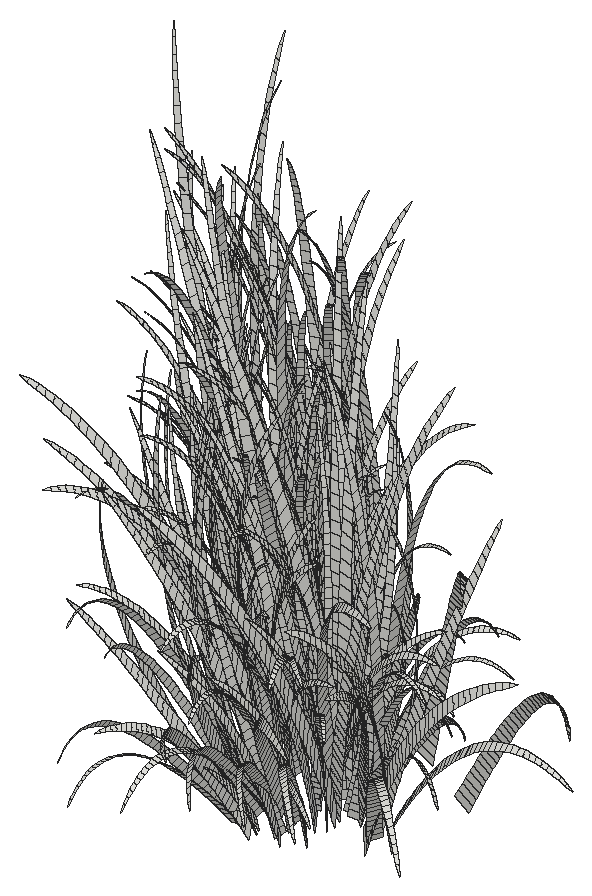
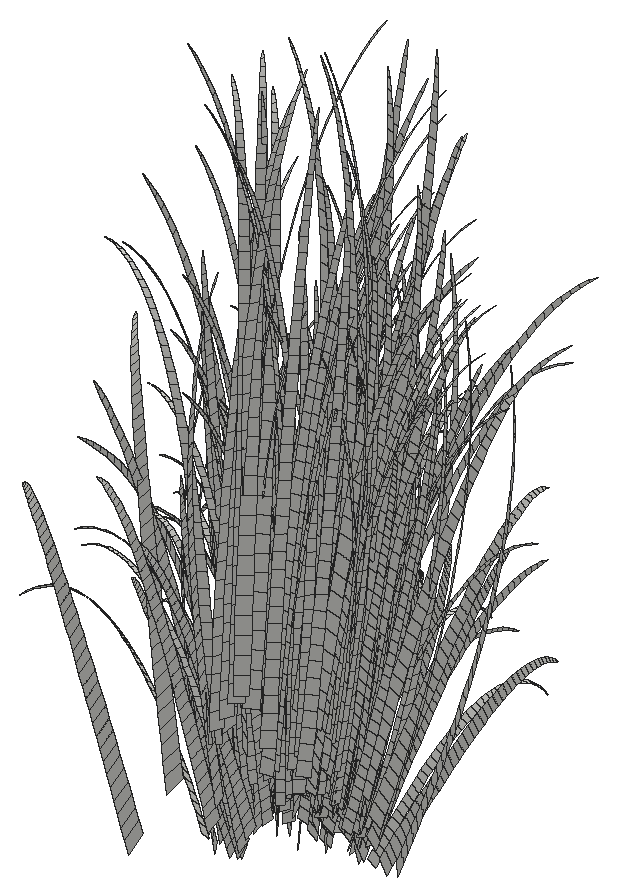
# SketchUp Ruby script. Lengths in inches.
U = 1.inch
M = Sketchup.active_model
def pt(a) = Geom::Point3d.new(a.map { |v| v * U })
def face(e, loops, mat)
  f = e.add_face(loops[0].map { |a| pt(a) })
  loops[1..].each { |l| e.add_face(l.map { |a| pt(a) }).erase! }
  f.material = f.back_material = mat if mat
  f
end
# faces: each face lists its corners as indices into pts; further lists are holes
def faces(e, pts, list, mat = nil) = list.each { |f| face(e, (f[0].is_a?(Array) ? f : [f]).map { |l| l.map { |i| pts[i] } }, mat) }
# xy, xz, yz: faces in a plane at the given z, y or x. An outline is a flat list of corners, or four numbers for a rectangle; further outlines are holes
def ring(l) = l.size == 4 ? [[l[0], l[1]], [l[2], l[1]], [l[2], l[3]], [l[0], l[3]]] : l.each_slice(2).to_a
def flat(e, list, mat, &to3) = list.each { |f| face(e, (f[0].is_a?(Array) ? f : [f]).map { |l| ring(l).map { |u, v| to3.(u, v) } }, mat) }
def xy(e, z, list, mat = nil) = flat(e, list, mat) { |x, y| [x, y, z] }
def xz(e, y, list, mat = nil) = flat(e, list, mat) { |x, z| [x, y, z] }
def yz(e, x, list, mat = nil) = flat(e, list, mat) { |y, z| [x, y, z] }
def lines(e, pts, list) = list.each { |a, b| e.add_line(pt(pts[a]), pt(pts[b])) }
# prism: a flat outline (further loops are holes) pulled along v
def prism(e, loops, v, mat = nil)
  f = face(e, loops, mat); d = Geom::Vector3d.new(v.map { |x| x * U })
  f.pushpull(f.normal.samedirection?(d) ? d.length : -d.length)
end
def box(e, o, s, mat = nil) = prism(e, [[o, [o[0] + s[0], o[1], o[2]], [o[0] + s[0], o[1] + s[1], o[2]], [o[0], o[1] + s[1], o[2]]]], [0, 0, s[2]], mat)
def at(x, y, z, deg = 0) = Geom::Transformation.translation(pt([x, y, z])) * Geom::Transformation.rotation(ORIGIN, Z_AXIS, deg.degrees)
def axes(o, x, y, z) = Geom::Transformation.new([*x, 0, *y, 0, *z, 0, *pt(o).to_a, 1])
def part(name) = M.definitions.add(name)
# library, detail: a bought-in or finely detailed component or shape, given as its bounding box
def library(name, o, s) = part(name).tap { |d| box(d.entities, o, s) }
def detail(e, o, s) = box(e.add_group.entities, o, s)
def put(e, d, t, mat = nil) = e.add_instance(d, t).tap { |i| i.material = mat if mat }
def group(e, t, mat = nil) = e.add_group.tap { |g| g.transformation = t; g.material = mat if mat }.entities
root = M.entities
c1 = part("fur_instance\#8")
p = [[-0.25,1.49,0.03],[0.25,-1.49,-0.03],[0.44,-1.47,1.51],[-0.05,1.47,1.57],[0.65,-1.44,3.05],[0.16,1.45,3.11],
  [0.86,-1.42,4.59],[0.38,1.44,4.65],[1.1,-1.39,6.13],[0.62,1.43,6.18],[1.34,-1.35,7.66],[0.875,1.42,7.72],
  [1.6,-1.32,9.19],[1.14,1.41,9.25],[1.88,-1.28,10.72],[1.43,1.41,10.78],[2.18,-1.24,12.25],[1.73,1.41,12.3],
  [2.49,-1.19,13.77],[2.05,1.41,13.82],[2.83,-1.15,15.29],[2.4,1.41,15.34],[3.18,-1.09,16.8],[2.76,1.42,16.85],
  [3.56,-1.03,18.31],[3.14,1.43,18.35],[3.96,-0.97,19.81],[3.55,1.44,19.85],[4.38,-0.91,21.3],[3.99,1.46,21.35],
  [4.84,-0.83,22.78],[4.45,1.48,22.83],[5.32,-0.76,24.26],[4.93,1.51,24.31],[5.82,-0.67,25.73],[5.45,1.54,25.77],
  [6.36,-0.59,27.18],[6,1.57,27.23],[6.93,-0.49,28.625],[6.58,1.61,28.67],[7.54,-0.39,30.05],[7.19,1.66,30.1],
  [8.18,-0.28,31.47],[7.84,1.71,31.51],[8.85,-0.16,32.86],[8.53,1.77,32.9],[9.57,-0.04,34.24],[9.25,1.83,34.27],
  [10.32,0.09,35.59],[10.02,1.9,35.625],[11.12,0.23,36.92],[10.82,1.97,36.95],[11.95,0.38,38.22],[11.67,2.06,38.25],
  [12.84,0.54,39.49],[12.57,2.14,39.52],[13.76,0.71,40.73],[13.51,2.24,40.76],[14.73,0.89,41.93],[14.49,2.34,41.95],
  [15.75,1.08,43.09],[15.52,2.45,43.11],[16.82,1.28,44.2],[16.6,2.5625,44.23],[17.93,1.5,45.27],[17.73,2.68,45.29],
  [19.08,1.73,46.28],[18.9,2.81,46.3],[20.29,1.97,47.24],[20.125,2.93,47.26],[21.53,2.22,48.13],[21.39,3.0625,48.15],
  [22.82,2.5,48.96],[22.7,3.1875,48.98],[24.14,2.8125,49.72],[24.06,3.3,49.73],[25.48,3.27,50.41]]
faces(c1.entities,p,[[0,1,2,3],[3,2,4,5],[5,4,6,7],[7,6,8,9],[9,8,10,11],[11,10,12,13],[13,12,14,15],[15,14,16,17],
  [17,16,18,19],[19,18,20,21],[21,20,22,23],[23,22,24,25],[25,24,26,27],[27,26,28,29],[29,28,30,31],[31,30,32,33],
  [33,32,34,35],[35,34,36,37],[37,36,38,39],[39,38,40,41],[41,40,42,43],[43,42,44,45],[45,44,46,47],[47,46,48,49],
  [49,48,50,51],[51,50,52,53],[53,52,54,55],[55,54,56,57],[57,56,58,59],[59,58,60,61],[61,60,62,63],[63,62,64,65],
  [65,64,66,67],[67,66,68,69],[69,68,70,71],[71,70,72,73],[73,72,74,75],[75,74,76]])
put(root,c1,axes([431.76,47.1,10.74],[0.15269,-0.07243,-0.24019],[0.13551,0.04613,0.26977],[-0.00773,-0.17522,0.28049]))
put(root,c1,axes([432.66,47.29,11.42],[-0.04322,-0.08103,-0.33227],[0.19342,-0.01502,-0.11763],[0.02265,-0.17179,0.27415]))
put(root,c1,axes([435.625,48.22,12.1],[-0.23798,-0.07441,0.13592],[0.01899,-0.11962,-0.43721],[0.10286,-0.20447,0.35918]))
put(root,c1,axes([432.39,47.27,11.41],[0.10158,-0.06914,-0.32205],[0.1701,0.0448,0.14301],[0.02265,-0.17174,0.27406]))
put(root,c1,axes([433.5,47.51,11.9],[0.19478,-0.02841,-0.30734],[0.1247,0.10642,0.29017],[0.06226,-0.20052,0.32988]))
put(root,c1,axes([431.09,47.14,10.46],[-0.02123,-0.06781,-0.31584],[0.17417,-0.05199,-0.00113],[-0.03366,-0.14772,0.24534]))
put(root,c1,axes([431.86,47.27,11.5],[0.19045,-0.03751,-0.06848],[0.03839,0.07261,0.33686],[-0.00736,-0.16676,0.26694]))
put(root,c1,axes([430.1,48.17,13.18],[0.03417,-0.12525,-0.29157],[0.20378,-0.0224,0.09589],[-0.03382,-0.15429,0.3542]))
put(root,c1,axes([433.28,48.3125,13.9],[-0.04153,-0.12718,-0.27595],[0.20481,-0.00989,-0.14624],[0.04417,-0.15922,0.36205]))
put(root,c1,axes([434.15,47.63,11.49],[0.10305,-0.05896,-0.3685],[0.16571,0.09891,0.06527],[0.08407,-0.16713,0.29358]))
put(root,c1,axes([430.21,47.49,10.73],[0.04168,-0.09258,-0.28201],[0.16554,-0.04371,0.15063],[-0.06017,-0.13932,0.24891]))
put(root,c1,axes([433.3125,47.64,12.03],[0.00165,-0.10984,-0.26082],[0.18149,0.01453,-0.07449],[0.03836,-0.13829,0.31445]))
put(root,c1,axes([433.15,47.38,11.42],[0.09702,-0.05494,-0.31246],[0.152,0.06601,0.10474],[0.04854,-0.15634,0.25719]))
put(root,c1,axes([433.41,47.54,11.92],[-0.19796,-0.00213,0.19119],[-0.0584,-0.09827,-0.32515],[0.05556,-0.17894,0.29438]))
put(root,c1,axes([431.97,48.57,15.22],[-0.18897,-0.07724,-0.16578],[0.14014,-0.11074,-0.30364],[0.02044,-0.18069,0.39971]))
put(root,c1,axes([432.17,48.16,14.25],[-0.25079,-0.01126,0.01167],[0.02691,-0.14432,-0.37072],[0.02191,-0.19373,0.42855]))
put(root,c1,axes([432.21,47.14,10.9],[-0.13424,-0.03889,-0.12787],[0.08866,-0.05443,-0.25596],[0.01839,-0.13945,0.22254]))
put(root,c1,axes([432.43,47.8125,13.16],[-0.22603,-0.01056,0.00948],[0.02497,-0.13008,-0.33426],[0.01976,-0.17466,0.38636]))
put(root,c1,axes([430.39,48.6,14.52],[0.00591,-0.15376,-0.2335],[0.21361,-0.03099,0.04882],[-0.02765,-0.13326,0.41924]))
put(root,c1,axes([434.61,48.46,12.95],[0.01148,-0.14011,-0.26001],[0.19146,0.05137,-0.16224],[0.08794,-0.13547,0.35942]))
put(root,c1,axes([437.57,49.37,11.02],[-0.15559,-0.16713,0.03304],[0.11706,-0.06849,-0.43118],[0.15185,-0.15167,0.34426]))
put(root,c1,axes([432,47.07,10.67],[0.1143,0.07759,0.29786],[-0.18253,0.04472,0.24081],[0.02462,-0.18668,0.29791]))
put(root,c1,axes([433.4,47.26,10.53],[-0.14554,-0.04613,0.08103],[0.01279,-0.07284,-0.26823],[0.06295,-0.12513,0.21981]))
put(root,c1,axes([430.62,47.75,11.82],[0.0606,-0.10906,-0.18612],[0.14677,-0.00638,0.15494],[-0.04628,-0.11412,0.28007]))
put(root,c1,axes([429.03,48.05,11.3125],[0.18766,-0.05407,0.15304],[-0.0375,0.10124,0.3241],[-0.06745,-0.15619,0.27904]))
put(root,c1,axes([430.98,47.34,11.42],[0.11054,0.06076,0.32124],[-0.18174,0.06569,0.1961],[-0.00805,-0.18258,0.29226]))
put(root,c1,axes([437.17,48.9375,11.01],[0.10396,-0.07911,-0.43973],[0.18772,0.13868,-0.01375],[0.12911,-0.17813,0.34745]))
put(root,c1,axes([433.3,49.16,15.93],[0.14666,-0.13638,-0.25039],[0.18844,0.10867,0.09026],[0.03514,-0.1508,0.47019]))
put(root,c1,axes([431.92,48.5625,14.4],[-0.00485,-0.13574,-0.20923],[0.19174,-0.01245,-0.03687],[0.01079,-0.12284,0.3739]))
put(root,c1,axes([432.63,47.67,12.82],[0.22137,0.04305,0.07377],[-0.08148,0.12835,0.33894],[0.02049,-0.18118,0.40078]))
put(root,c1,axes([431.93,47.04,10.48],[-0.16406,0.03446,0.0684],[-0.03839,-0.06194,-0.29017],[-0.00638,-0.14462,0.2315]))
put(root,c1,axes([433.46,48.73,14.72],[-0.14817,-0.12463,-0.07303],[0.15181,-0.10509,-0.22784],[0.04979,-0.1294,0.42509]))
put(root,c1,axes([435.0625,48.6,13.56],[0.20792,-0.04098,-0.29203],[0.11115,0.15527,0.21492],[0.07916,-0.17504,0.42246]))
put(root,c1,axes([434.34,47.84,10.5625],[-0.12758,-0.07753,0.0557],[0.04435,-0.06394,-0.27127],[0.08127,-0.11212,0.2187]))
put(root,c1,axes([433.4,47.25,10.62],[-0.08929,0.05587,0.30832],[-0.15159,-0.06244,-0.09121],[0.04736,-0.15254,0.25094]))
put(root,c1,axes([434.62,48.13,11.27],[-0.14977,-0.06071,0.14936],[0.00439,-0.0935,-0.26844],[0.09015,-0.12438,0.2426]))
put(root,c1,axes([433.91,48.96,14.34],[-0.02184,-0.15888,-0.15748],[0.19236,-0.00034,-0.15603],[0.06127,-0.11125,0.39683]))
put(root,c1,axes([433.46,49.32,15.85],[-0.16708,-0.12567,-0.06302],[0.15179,-0.11958,-0.24667],[0.05298,-0.1377,0.45233]))
put(root,c1,axes([433.67,48.35,13.34],[0.12346,-0.06874,-0.2664],[0.133,0.10274,0.08323],[0.06093,-0.13474,0.32518]))
put(root,c1,axes([433.8,47.58,10.99],[0.10797,-0.02278,-0.25368],[0.09924,0.08349,0.12145],[0.06318,-0.1256,0.22064]))
put(root,c1,axes([432.49,48.67,14.4],[-0.10701,-0.11213,-0.12442],[0.15233,-0.07687,-0.16606],[0.02739,-0.11756,0.36656]))
put(root,c1,axes([431.63,47.8125,12.75],[-0.15193,-0.01941,-0.09588],[0.0644,-0.09304,-0.22233],[-0.00624,-0.12588,0.27933]))
put(root,c1,axes([431.27,47.66,12.25],[0.16669,-0.01734,0.08094],[-0.02966,0.10281,0.23812],[-0.02771,-0.12642,0.29024]))
put(root,c1,axes([434.93,48.45,11.33],[-0.13012,-0.10057,0.10963],[0.04873,-0.08061,-0.28847],[0.10836,-0.10823,0.24566]))
put(root,c1,axes([433.22,47.85,12.71],[0.19476,0.01919,-0.07142],[-0.00771,0.11743,0.2824],[0.0412,-0.14851,0.33769]))
put(root,c1,axes([432.78,47.91,12.75],[0.12624,-0.07118,-0.14847],[0.09892,0.09301,0.09957],[0.0236,-0.10128,0.3158]))
put(root,c1,axes([433.99,48.42,12.36],[-0.08522,-0.11751,-0.02593],[0.11177,-0.04315,-0.23298],[0.08081,-0.09116,0.27707]))
put(root,c1,axes([434.77,48.47,12.62],[-0.18644,-0.03104,0.19118],[-0.0143,-0.14214,-0.22961],[0.08573,-0.13206,0.3504]))
put(root,c1,axes([433.64,47.6,11.46],[0.15494,0.00054,-0.15254],[0.03594,0.10834,0.19122],[0.0534,-0.11809,0.285]))
put(root,c1,axes([431.47,47.46,11.95],[0.12347,0.06755,0.21237],[-0.14396,0.08585,0.17984],[-0.00718,-0.14468,0.32104]))
put(root,c1,axes([434.66,49.22,13.59],[-0.12334,-0.12969,0.01714],[0.11431,-0.07492,-0.27994],[0.09668,-0.10907,0.33149]))
put(root,c1,axes([435.3,49.05,14.4],[-0.21667,0.03837,0.29524],[-0.10928,-0.16078,-0.2283],[0.08148,-0.18018,0.43484]))
put(root,c1,axes([434.62,49.91,15.73],[-0.1604,-0.13739,-0.02167],[0.15059,-0.11716,-0.25101],[0.06963,-0.12643,0.45099]))
put(root,c1,axes([435.875,49.34,11.53],[-0.06626,-0.1567,-0.04431],[0.12258,-0.00555,-0.33309],[0.13287,-0.09611,0.2699]))
put(root,c1,axes([434.39,48.39,11.73],[0.05454,-0.09644,-0.21571],[0.13016,0.08062,-0.0942],[0.08114,-0.09154,0.27821]))
put(root,c1,axes([432.15,48.56,14.18],[-0.16225,-0.04777,-0.05886],[0.07812,-0.11873,-0.19059],[0.01013,-0.11533,0.35104]))
put(root,c1,axes([432.34,47.97,12.95],[0.15315,-0.04031,-0.07636],[0.04669,0.1064,0.16007],[0.009,-0.10254,0.31211]))
put(root,c1,axes([432.34,47.68,12.51],[-0.13701,0.06738,0.19305],[-0.11347,-0.07671,-0.17654],[0.01546,-0.13663,0.30225]))
put(root,c1,axes([431.43,47.42,11.68],[0.07036,0.07691,0.22077],[-0.15002,0.05652,0.10186],[-0.00627,-0.1264,0.28049]))
put(root,c1,axes([432.17,49.22,15.2],[0.10618,-0.13596,-0.12929],[0.15853,0.08066,0.0353],[0.01505,-0.09183,0.40695]))
put(root,c1,axes([433.66,48.32,13.57],[-0.14966,0.06135,0.2769],[-0.12806,-0.11932,-0.12286],[0.06613,-0.14624,0.35295]))
put(root,c1,axes([430.94,50.92,18.59],[0.02992,-0.20268,-0.17218],[0.24479,0.00013,0.02509],[-0.00825,-0.12029,0.52424]))
put(root,c1,axes([433.03,47.96,12.9],[0.16263,0.05278,0.0273],[-0.0671,0.09353,0.2615],[0.03718,-0.13404,0.3048]))
put(root,c1,axes([433.11,49.14,14.42],[0.0438,-0.14683,-0.11127],[0.16937,0.03664,-0.05087],[0.03107,-0.07683,0.37846]))
put(root,c1,axes([433.9,48.625,14.72],[-0.10088,0.13062,0.3695],[-0.228,-0.07812,-0.04804],[0.0527,-0.18996,0.43195]))
put(root,c1,axes([431.79,47.4375,11.82],[-0.02267,0.09523,0.24051],[-0.16406,0.00552,-0.03477],[-0.00627,-0.12634,0.28034]))
put(root,c1,axes([433.29,48.26,12.84],[-0.14955,-0.02951,0.08847],[0.01953,-0.12021,-0.14832],[0.04773,-0.08667,0.30915]))
put(root,c1,axes([430.65,48,12.64],[0.10535,0.0488,0.23666],[-0.12967,0.10407,0.09442],[-0.04869,-0.12008,0.29468]))
put(root,c1,axes([431.88,47.72,12.61],[0.01737,0.09262,0.24572],[-0.16736,0.02852,0.02395],[-0.00637,-0.12835,0.28481]))
put(root,c1,axes([431.48,50.52,16.99],[0.04164,-0.17352,-0.14577],[0.20763,0.01338,0.03275],[-0.00709,-0.10329,0.45016]))
put(root,c1,axes([430.89,48.21,13.27],[0.16477,0.01322,0.09468],[-0.05646,0.12716,0.16983],[-0.02254,-0.10862,0.34171]))
put(root,c1,axes([429.36,48.78,12.94],[0.15549,-0.01208,0.20833],[-0.06905,0.13306,0.17126],[-0.07165,-0.11508,0.31313]))
put(root,c1,axes([431.12,50.11,15.96],[-0.00432,-0.15952,-0.128],[0.19173,-0.03266,0.04648],[-0.02798,-0.08806,0.41192]))
put(root,c1,axes([433.14,48.63,13.78],[-0.16995,0.00239,0.1052],[-0.0155,-0.13112,-0.16118],[0.04006,-0.1041,0.34197]))
put(root,c1,axes([431.98,49.48,15.19],[-0.13495,-0.09194,-0.07228],[0.12419,-0.11921,-0.10694],[0.00432,-0.08968,0.38985]))
put(root,c1,axes([436.74,49.67,12.4375],[-0.14869,0.01051,0.38769],[-0.10168,-0.16677,-0.09879],[0.14048,-0.14032,0.31849]))
put(root,c1,axes([431.08,48.64,13.82],[0.1599,-0.01285,0.09328],[-0.0299,0.12534,0.15874],[-0.03604,-0.09723,0.32437]))
put(root,c1,axes([431.8125,49.04,14.28],[0.14874,-0.07113,-0.04632],[0.06911,0.1145,0.10604],[-0.00549,-0.08,0.34865]))
put(root,c1,axes([432.84,49.62,14.37],[-0.04201,-0.14205,-0.02716],[0.15521,-0.03808,-0.10788],[0.03986,-0.0584,0.35377]))
put(root,c1,axes([435.33,48.49,11.86],[0.07572,0.13089,0.20219],[-0.15985,-0.01369,0.30106],[0.10643,-0.14683,0.2864]))
put(root,c1,axes([431.74,48.33,13.59],[0.12885,0.05972,0.11755],[-0.10424,0.10176,0.1411],[-0.00603,-0.1057,0.32265]))
put(root,c1,axes([435.05,48.86,12.375],[0.16454,0.02683,-0.22071],[0.01929,0.1451,0.16624],[0.09525,-0.10745,0.32659]))
put(root,c1,axes([433.875,51.45,18.55],[0.143,-0.17445,-0.17187],[0.20045,0.12222,-0.01071],[0.04373,-0.10813,0.53269]))
put(root,c1,axes([432.6,49.87,15.11],[0.11075,-0.11944,-0.11937],[0.13443,0.0987,-0.0216],[0.03784,-0.07056,0.38011]))
put(root,c1,axes([434.76,51.77,17.44],[-0.03736,-0.20284,-0.08426],[0.21276,-0.01244,-0.24024],[0.09664,-0.09898,0.46456]))
put(root,c1,axes([435.17,49.61,12.74],[0.12005,-0.06141,-0.26447],[0.09556,0.14151,-0.0324],[0.10376,-0.08664,0.31771]))
put(root,c1,axes([431.75,50,16.0625],[-0.18618,-0.03996,-0.02577],[0.06509,-0.15689,-0.1364],[0.00464,-0.09644,0.41925]))
put(root,c1,axes([431.84,50.92,18.87],[0.24074,-0.08114,-0.0797],[0.07823,0.19128,0.15934],[0.00596,-0.12377,0.53808]))
put(root,c1,axes([431.05,49.69,14.16],[-0.04654,-0.13259,-0.03011],[0.14978,-0.05997,0.02545],[-0.01873,-0.03986,0.3514]))
put(root,c1,axes([431.19,48.51,14.47],[-0.06192,0.14505,0.21697],[-0.19671,-0.02273,-0.07174],[-0.0075,-0.13152,0.40147]))
put(root,c1,axes([435.54,49.66,11.39],[0.06859,-0.09014,-0.25373],[0.09618,0.12505,-0.16822],[0.12923,-0.06487,0.24688]))
put(root,c1,axes([431.79,50.08,15.77],[-0.1296,-0.11177,-0.03307],[0.13714,-0.12794,-0.0397],[-0.00189,-0.06022,0.41924]))
put(root,c1,axes([434.78,52.05,18.92],[-0.20857,-0.13075,0.08955],[0.12369,-0.16885,-0.26752],[0.09431,-0.12712,0.50956]))
put(root,c1,axes([435.6,48.88,13.02],[-0.00332,0.15612,0.27725],[-0.2105,-0.04955,0.19049],[0.09652,-0.14869,0.3945]))
put(root,c1,axes([436.65,48.89,10.72],[0.1674,0.12348,-0.15342],[-0.05527,0.10723,0.36025],[0.13749,-0.13733,0.3117]))
put(root,c1,axes([432.21,49.37,16.375],[-0.15736,0.12863,0.21317],[-0.17096,-0.10355,-0.14422],[0.01307,-0.14881,0.45294]))
put(root,c1,axes([435.76,49.11,13.61],[0.15805,0.15051,0.05502],[-0.15454,0.08321,0.34889],[0.10135,-0.15612,0.41421]))
put(root,c1,axes([434.91,49.05,12.15],[0.14109,0.00407,-0.23949],[0.03377,0.14579,0.07817],[0.0981,-0.08192,0.30039]))
put(root,c1,axes([432.26,48.47,13.64],[-0.14242,0.06423,0.07833],[-0.06984,-0.11466,-0.07925],[0.01251,-0.07634,0.33832]))
put(root,c1,axes([430.25,51.97,19.24],[0.18706,-0.15692,-0.05371],[0.1539,0.13296,0.16341],[-0.03534,-0.11123,0.5203]))
put(root,c1,axes([435.59,49.67,11.95],[0.12063,-0.06515,-0.25144],[0.08341,0.14829,-0.07405],[0.10987,-0.06634,0.31554]))
put(root,c1,axes([434.72,49.93,12.05],[0.0496,-0.12974,-0.10453],[0.11629,0.07093,-0.20268],[0.09864,-0.03996,0.27723]))
put(root,c1,axes([437.55,51.85,13.8],[0.04979,-0.1895,-0.18773],[0.18438,0.09265,-0.2851],[0.14308,-0.0864,0.41092]))
put(root,c1,axes([435.55,49.16,12.3],[-0.10089,0.09227,0.28247],[-0.13958,-0.12254,0.05217],[0.09902,-0.11171,0.33951]))
put(root,c1,axes([431.42,48.61,14.06],[0.0286,0.11518,0.18982],[-0.16763,0.04809,-0.0018],[-0.022,-0.10604,0.33361]))
put(root,c1,axes([434.94,49.47,14.93],[-0.03936,0.14543,0.30601],[-0.20696,-0.07562,0.14027],[0.09659,-0.14879,0.39477]))
put(root,c1,axes([433.68,52.4375,19.64],[0.12423,-0.19532,-0.16493],[0.21975,0.1108,-0.06089],[0.05484,-0.10226,0.55089]))
put(root,c1,axes([432.39,49.03,15.04],[-0.07914,0.12591,0.21103],[-0.17333,-0.05924,-0.02394],[0.02804,-0.12033,0.37519]))
put(root,c1,axes([434.26,48.8,12.54],[-0.09743,0.06774,0.23139],[-0.09599,-0.11967,0.05358],[0.09249,-0.07723,0.28321]))
put(root,c1,axes([432.11,50.38,15.06],[-0.07961,-0.13689,0.01423],[0.15313,-0.0843,-0.034],[0.01219,-0.0383,0.38556]))
put(root,c1,axes([433.5,50.03,14.03],[0.10839,-0.11453,-0.08174],[0.11795,0.10157,-0.07097],[0.04416,-0.04194,0.35588]))
put(root,c1,axes([433.65,49.64,13.78],[-0.14662,-0.03521,0.15792],[0.02351,-0.14317,-0.07806],[0.07228,-0.05609,0.32502]))
put(root,c1,axes([432.16,50.29,14.67],[-0.07124,-0.13476,0.02236],[0.14958,-0.07747,-0.02272],[0.00941,-0.03103,0.37011]))
put(root,c1,axes([432.61,52.16,19.21],[-0.1863,-0.12854,0.00057],[0.15019,-0.16226,-0.16735],[0.0425,-0.10509,0.5177]))
put(root,c1,axes([435.8125,49.2,11.44],[-0.0662,0.08995,0.30205],[-0.12202,-0.12772,0.14438],[0.13238,-0.09575,0.2689]))
put(root,c1,axes([432.51,50.67,15.68],[-0.12883,-0.11449,0.01319],[0.1336,-0.12723,-0.04151],[0.01291,-0.04776,0.41418]))
put(root,c1,axes([434.29,52.55,18.44],[-0.02329,-0.21903,-0.03429],[0.23378,-0.02287,-0.15724],[0.06291,-0.07396,0.52011]))
put(root,c1,axes([435.34,50.33,12.98],[-0.14894,-0.04461,0.24591],[0.01234,-0.15892,-0.10432],[0.11196,-0.06761,0.32156]))
put(root,c1,axes([430.06,50.07,13.59],[0.09225,-0.12894,0.11038],[0.10291,0.0771,0.12838],[-0.07903,-0.02356,0.31361]))
put(root,c1,axes([434.88,52.47,17.66],[-0.02212,-0.21398,-0.03391],[0.22838,-0.02174,-0.15347],[0.06144,-0.07223,0.50797]))
put(root,c1,axes([431,49,13.87],[0.13738,0.0414,0.0972],[-0.07592,0.13055,0.05523],[-0.03104,-0.06782,0.34028]))
put(root,c1,axes([435.27,50.18,10.85],[-0.03175,-0.14429,0.13902],[0.10175,-0.04851,-0.23869],[0.11949,-0.01479,0.22844]))
put(root,c1,axes([432.11,50.79,15.46],[-0.07772,-0.14595,0.01956],[0.16231,-0.0838,-0.0308],[0.01178,-0.03674,0.40206]))
put(root,c1,axes([431.69,50.12,15.08],[0.16142,-0.07143,-0.01571],[0.0631,0.13884,0.04506],[-0.00507,-0.05525,0.3852]))
put(root,c1,axes([431.24,50.89,16.24],[-0.13872,-0.10688,-0.05008],[0.13478,-0.14007,-0.01499],[-0.01621,-0.05768,0.43132]))
put(root,c1,axes([432.62,49.88,14.34],[0.13914,-0.08385,-0.03496],[0.08075,0.12335,-0.00894],[0.01158,-0.03859,0.35924]))
put(root,c1,axes([435.61,49.2,11.62],[-0.05491,0.09737,0.28251],[-0.12379,-0.11722,0.16383],[0.12913,-0.0934,0.26231]))
put(root,c1,axes([432.93,50.25,14.21],[-0.08777,-0.12311,0.07978],[0.13105,-0.09185,-0.0647],[0.04014,-0.02395,0.34954]))
put(root,c1,axes([433.32,50.91,15.26],[0.07494,-0.15978,-0.03962],[0.16264,0.06715,-0.11216],[0.04856,-0.037,0.39794]))
put(root,c1,axes([432.31,49.04,15.01],[-0.1422,0.11091,0.11586],[-0.12628,-0.11191,-0.06649],[0.015,-0.09153,0.40561]))
put(root,c1,axes([433.77,52.56,19.32],[0.15717,-0.16888,-0.16909],[0.19008,0.14007,-0.03029],[0.05359,-0.09991,0.53827]))
put(root,c1,axes([432.32,49.25,14.46],[-0.14765,0.06695,0.09599],[-0.07527,-0.12279,-0.06548],[0.02169,-0.07701,0.35566]))
put(root,c1,axes([430.95,49.43,15.96],[0.0038,0.14954,0.23139],[-0.20994,0.03733,-0.03743],[-0.02717,-0.13094,0.41195]))
put(root,c1,axes([430.73,49.84,17.43],[-0.04308,0.17847,0.273],[-0.24701,-0.00413,-0.05166],[-0.00912,-0.15991,0.48813]))
put(root,c1,axes([434.01,50.1,17.19],[0.19083,0.13184,0.05677],[-0.15811,0.13743,0.27367],[0.05817,-0.15117,0.49659]))
put(root,c1,axes([436.14,50.92,11.04],[-0.09134,-0.12785,0.22656],[0.07697,-0.11104,-0.22116],[0.1384,-0.04262,0.25929]))
put(root,c1,axes([431.125,51.03,15.41],[-0.00822,-0.16722,0.01164],[0.17876,-0.02595,0.03382],[-0.01925,-0.0303,0.40131]))
put(root,c1,axes([431.57,49.78,14.64],[0.16373,-0.03857,0.00921],[0.02397,0.14494,0.04432],[-0.01107,-0.05099,0.36849]))
put(root,c1,axes([434.72,50.2,14.23],[0.16409,-0.04331,-0.20606],[0.05728,0.16704,-0.00737],[0.08461,-0.06565,0.38043]))
put(root,c1,axes([434.59,48.89,11.95],[0.12216,0.08749,-0.1288],[-0.05725,0.10364,0.19567],[0.09123,-0.07618,0.27934]))
put(root,c1,axes([432.91,50.125,14.71],[0.1463,-0.07615,-0.10409],[0.07711,0.13848,-0.04067],[0.04559,-0.04329,0.3674]))
put(root,c1,axes([435.89,51.27,16.125],[0.20327,-0.05604,-0.25675],[0.08292,0.19878,0.03195],[0.09822,-0.10059,0.47212]))
put(root,c1,axes([432.7,51.59,18.4],[-0.22223,-0.05187,0.06437],[0.06185,-0.19269,-0.14793],[0.04097,-0.1013,0.49904]))
put(root,c1,axes([430.84,48.77,13.67],[0.09089,0.09523,0.11248],[-0.12952,0.09997,0.00707],[-0.03129,-0.06837,0.34303]))
put(root,c1,axes([431,49.53,15.09],[0.15043,0.06237,0.10618],[-0.10193,0.14112,0.07332],[-0.02651,-0.08344,0.39031]))
put(root,c1,axes([430.88,51.25,15.99],[-0.09202,-0.14419,-0.02135],[0.16494,-0.10399,0.03603],[-0.02333,-0.03794,0.42396]))
put(root,c1,axes([434.61,49.42,12.39],[-0.11286,0.04976,0.22948],[-0.06771,-0.13658,0.05175],[0.0986,-0.05954,0.28318]))
put(root,c1,axes([431.72,51.32,16.46],[0.12208,-0.15013,-0.02869],[0.15272,0.10311,-0.03034],[0.01381,-0.04339,0.43679]))
put(root,c1,axes([435.0625,50.09,13.15],[-0.14023,0.01888,0.26296],[-0.04453,-0.1614,-0.00292],[0.11023,-0.06656,0.31656]))
put(root,c1,axes([434.48,49.27,13.65],[0.13121,0.11551,-0.02739],[-0.11587,0.10209,0.2018],[0.06808,-0.09176,0.36783]))
put(root,c1,axes([434.95,50.51,15.77],[0.20769,0.04966,-0.15926],[-0.03101,0.17814,0.18526],[0.08167,-0.11008,0.44127]))
put(root,c1,axes([435.51,50.47,10.98],[0.068,-0.12804,-0.12081],[0.08818,0.09434,-0.26208],[0.12484,-0.01545,0.23865]))
put(root,c1,axes([435.13,50.4375,11.08],[0.06266,-0.1249,-0.10853],[0.0861,0.08678,-0.25374],[0.11938,-0.01478,0.22823]))
put(root,c1,axes([432.85,50.97,18.01],[0.23315,0.01342,-0.06471],[-0.02237,0.19719,0.15093],[0.03065,-0.10883,0.50265]))
put(root,c1,axes([432.41,50.78,14.78],[0.11708,-0.12342,-0.00631],[0.12225,0.10057,-0.03033],[0.0076,-0.02912,0.37804]))
put(root,c1,axes([433.56,50.63,15.57],[-0.18521,-0.02955,0.11381],[0.03239,-0.17376,-0.06029],[0.05035,-0.05919,0.41626]))
put(root,c1,axes([432.57,51.52,17.33],[-0.17633,-0.09809,0.01724],[0.1199,-0.16919,-0.04915],[0.01352,-0.05835,0.47546]))
put(root,c1,axes([432.4375,49.15,14.62],[0.0987,0.11897,0.05521],[-0.14378,0.08662,0.10909],[0.02282,-0.08103,0.37425]))
put(root,c1,axes([433.08,50.16,13.95],[0.13682,-0.07692,-0.07129],[0.07213,0.1295,-0.07116],[0.03936,-0.02349,0.34277]))
put(root,c1,axes([432.7,49.59,14.29],[0.15222,0.03642,-0.07852],[-0.03946,0.13914,0.07531],[0.03898,-0.05711,0.34597]))
put(root,c1,axes([431.58,49.03,14.09],[0.0055,0.12915,0.11043],[-0.15799,0.02454,-0.01796],[-0.01431,-0.07554,0.33727]))
put(root,c1,axes([435.67,49.6,12.66],[-0.06239,0.13265,0.23168],[-0.15342,-0.10065,0.1704],[0.112,-0.09352,0.34293]))
put(root,c1,axes([430.32,50.43,14.91],[0.1666,-0.05285,0.10887],[0.0248,0.15525,0.04679],[-0.05548,-0.04238,0.37888]))
put(root,c1,axes([429.86,50.92,16.81],[0.2061,-0.01344,0.1131],[-0.02793,0.18662,0.09605],[-0.05077,-0.08252,0.4557]))
put(root,c1,axes([435.32,51.71,13.82],[-0.06465,-0.16754,0.157],[0.14103,-0.07728,-0.22676],[0.11827,-0.02606,0.33858]))
put(root,c1,axes([433.95,49.46,14.6875],[0.10826,0.14171,0.01778],[-0.14869,0.07846,0.21324],[0.07154,-0.09642,0.38649]))
put(root,c1,axes([431.75,49.61,14.65],[-0.15853,0.06077,0.01255],[-0.05151,-0.13731,-0.04414],[-0.00488,-0.05314,0.37046]))
put(root,c1,axes([431.57,51.28,15.35],[0.10751,-0.14401,0.02773],[0.14274,0.0886,-0.01156],[-0.00773,-0.0245,0.39927]))
put(root,c1,axes([433.99,49.93,16.03],[0.10368,0.16194,0.09463],[-0.18699,0.06759,0.22582],[0.06767,-0.12287,0.43828]))
put(root,c1,axes([434.75,50.86,11.58],[0.04832,-0.14518,0.00787],[0.12065,0.04323,-0.22286],[0.09094,-0.00311,0.27632]))
put(root,c1,axes([433.61,49.24,13.84],[0.10539,0.11766,-0.04264],[-0.11395,0.08648,0.1779],[0.06944,-0.07112,0.33381]))
put(root,c1,axes([430.67,49.76,14.74],[0.13539,0.06511,0.11886],[-0.10233,0.13809,0.02305],[-0.04143,-0.06734,0.37184]))
put(root,c1,axes([431.12,49.32,15.46],[-0.0211,0.16438,0.13367],[-0.19675,0.00758,-0.04177],[-0.01791,-0.09455,0.42215]))
put(root,c1,axes([432.54,51.92,16.54],[-0.11995,-0.14094,0.03187],[0.15995,-0.12378,-0.02155],[0.01135,-0.03745,0.44662]))
put(root,c1,axes([429.74,51.31,18.33],[0.22597,0.02863,0.10796],[-0.07525,0.20019,0.13019],[-0.03474,-0.10937,0.51158]))
put(root,c1,axes([432.6,51.15,14.39],[-0.02615,-0.15514,0.08978],[0.1636,-0.03862,-0.04775],[0.02391,-0.00243,0.36067]))
put(root,c1,axes([434.9,50.22,12.625],[-0.13363,0.01209,0.24348],[-0.02341,-0.15821,0.02454],[0.10585,-0.04288,0.29749]))
put(root,c1,axes([433.68,50.71,13.98],[-0.12808,-0.08127,0.17105],[0.08472,-0.13879,-0.03962],[0.07069,-0.01437,0.33524]))
put(root,c1,axes([436.52,49.82,11.05],[0.04443,0.16095,0.1082],[-0.13761,-0.02397,0.33152],[0.13789,-0.09974,0.2801]))
put(root,c1,axes([437.02,50.48,11.11],[0.13942,0.04831,-0.34302],[0.00816,0.17572,0.1089],[0.15278,-0.07668,0.29185]))
put(root,c1,axes([433.4,50.98,13.23],[0.01848,-0.15029,0.09797],[0.14831,0.00119,-0.12824],[0.05045,0.01072,0.31409]))
put(root,c1,axes([431.86,52.57,16.91],[-0.03248,-0.18789,0.03246],[0.20264,-0.04691,-0.01246],[0.00277,-0.0305,0.45814]))
put(root,c1,axes([432.98,49.93,16.5],[0.1142,0.15271,0.07486],[-0.18421,0.10064,0.13224],[0.02836,-0.10071,0.46512]))
put(root,c1,axes([432.09,49.86,16.42],[-0.01068,0.1751,0.14296],[-0.21108,0.00073,0.04004],[0.01667,-0.10172,0.45077]))
put(root,c1,axes([431.07,50.26,17.94],[0.08928,0.17665,0.16183],[-0.22737,0.09539,0.05927],[-0.00818,-0.11915,0.51927]))
put(root,c1,axes([431.73,50.45,16.34],[-0.18895,0.06999,0.02245],[-0.05996,-0.16418,-0.04942],[-0.00199,-0.06326,0.44045]))
put(root,c1,axes([430.21,52.66,17.18],[0.12224,-0.1724,0.03147],[0.17004,0.09672,0.03094],[-0.02457,-0.03858,0.46994]))
put(root,c1,axes([435.69,51.62,12.54],[0.11573,-0.11352,-0.17299],[0.09518,0.13737,-0.20258],[0.11423,-0.02517,0.32701]))
put(root,c1,axes([438.54,53.125,11.35],[0.07286,-0.17069,-0.21842],[0.13329,0.1313,-0.33824],[0.176,-0.05419,0.32974]))
put(root,c1,axes([435.45,50.68,12.21],[0.14053,0.00256,-0.25431],[0.0115,0.16488,-0.00221],[0.11001,-0.04457,0.30917]))
put(root,c1,axes([434.4,50.83,12.29],[0.11365,-0.08796,-0.13302],[0.06535,0.12495,-0.18142],[0.09174,-0.00314,0.27875]))
put(root,c1,axes([430.53,50.26,14.32],[0.15146,0.01629,0.10652],[-0.04117,0.15418,-0.02273],[-0.05245,-0.03078,0.35407]))
put(root,c1,axes([431.58,53.26,18.3],[0.0752,-0.20516,0.02464],[0.21175,0.0536,-0.02901],[0.00304,-0.03339,0.50163]))
put(root,c1,axes([431.27,50.2,16.1875],[-0.02865,0.1632,0.13083],[-0.19416,0.00105,-0.04665],[-0.01776,-0.09378,0.4187]))
put(root,c1,axes([430.93,49.59,14.25],[-0.03907,0.14419,0.04289],[-0.15068,-0.00691,-0.10234],[-0.04404,-0.05511,0.34471]))
put(root,c1,axes([435.18,50.24,12.8],[0.13705,0.06092,-0.24143],[-0.03897,0.15511,0.08813],[0.11117,-0.04504,0.31244]))
put(root,c1,axes([432.38,49.57,14.3125],[-0.08483,0.12977,0.03637],[-0.13576,-0.06868,0.01436],[0.01015,-0.0438,0.35695]))
put(root,c1,axes([431.61,53.29,17.09],[0.00458,-0.19714,0.03462],[0.20895,-0.01368,-0.00104],[-0.00501,-0.02872,0.46671]))
